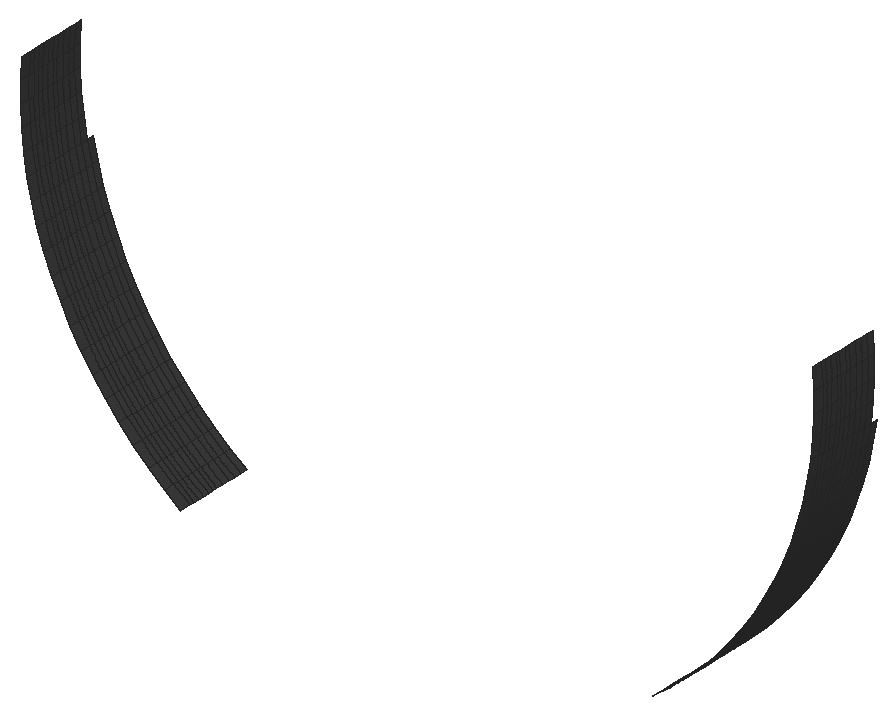
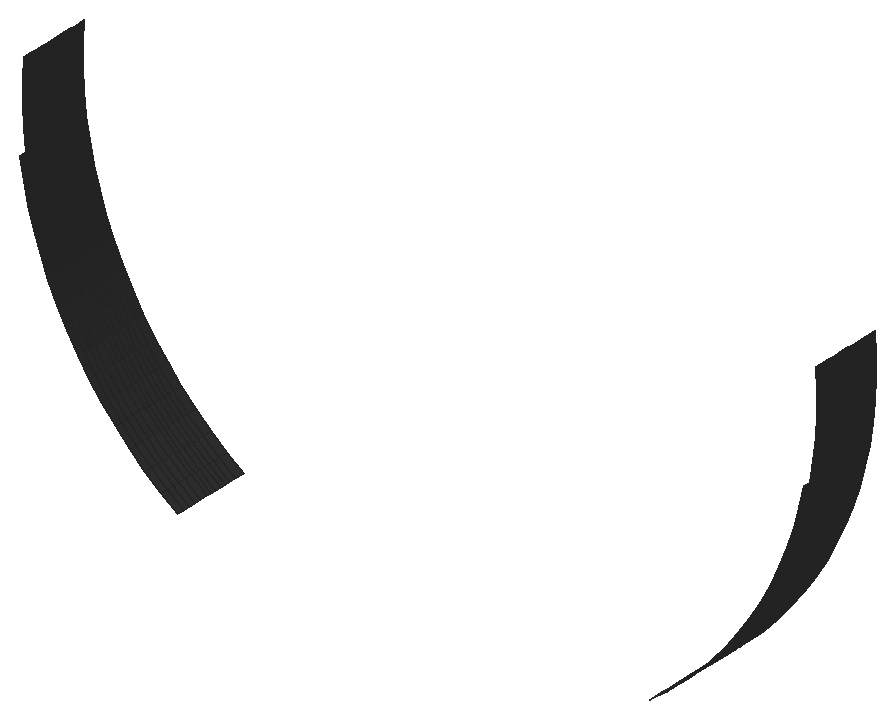
# SketchUp Ruby script. Lengths in inches.
U = 1.inch
M = Sketchup.active_model
def pt(a) = Geom::Point3d.new(a.map { |v| v * U })
def face(e, loops, mat)
  f = e.add_face(loops[0].map { |a| pt(a) })
  loops[1..].each { |l| e.add_face(l.map { |a| pt(a) }).erase! }
  f.material = f.back_material = mat if mat
  f
end
# faces: each face lists its corners as indices into pts; further lists are holes
def faces(e, pts, list, mat = nil) = list.each { |f| face(e, (f[0].is_a?(Array) ? f : [f]).map { |l| l.map { |i| pts[i] } }, mat) }
# xy, xz, yz: faces in a plane at the given z, y or x. An outline is a flat list of corners, or four numbers for a rectangle; further outlines are holes
def ring(l) = l.size == 4 ? [[l[0], l[1]], [l[2], l[1]], [l[2], l[3]], [l[0], l[3]]] : l.each_slice(2).to_a
def flat(e, list, mat, &to3) = list.each { |f| face(e, (f[0].is_a?(Array) ? f : [f]).map { |l| ring(l).map { |u, v| to3.(u, v) } }, mat) }
def xy(e, z, list, mat = nil) = flat(e, list, mat) { |x, y| [x, y, z] }
def xz(e, y, list, mat = nil) = flat(e, list, mat) { |x, z| [x, y, z] }
def yz(e, x, list, mat = nil) = flat(e, list, mat) { |y, z| [x, y, z] }
def lines(e, pts, list) = list.each { |a, b| e.add_line(pt(pts[a]), pt(pts[b])) }
# prism: a flat outline (further loops are holes) pulled along v
def prism(e, loops, v, mat = nil)
  f = face(e, loops, mat); d = Geom::Vector3d.new(v.map { |x| x * U })
  f.pushpull(f.normal.samedirection?(d) ? d.length : -d.length)
end
def box(e, o, s, mat = nil) = prism(e, [[o, [o[0] + s[0], o[1], o[2]], [o[0] + s[0], o[1] + s[1], o[2]], [o[0], o[1] + s[1], o[2]]]], [0, 0, s[2]], mat)
def at(x, y, z, deg = 0) = Geom::Transformation.translation(pt([x, y, z])) * Geom::Transformation.rotation(ORIGIN, Z_AXIS, deg.degrees)
def axes(o, x, y, z) = Geom::Transformation.new([*x, 0, *y, 0, *z, 0, *pt(o).to_a, 1])
def part(name) = M.definitions.add(name)
# library, detail: a bought-in or finely detailed component or shape, given as its bounding box
def library(name, o, s) = part(name).tap { |d| box(d.entities, o, s) }
def detail(e, o, s) = box(e.add_group.entities, o, s)
def put(e, d, t, mat = nil) = e.add_instance(d, t).tap { |i| i.material = mat if mat }
def group(e, t, mat = nil) = e.add_group.tap { |g| g.transformation = t; g.material = mat if mat }.entities
root = M.entities
M.materials.add("[Color M07]").color = [58, 58, 58]
yz(root,46.34,[[13.45,175.125,14.95,178.17],[14.95,175.125,15.8,178.17],[15.8,175.125,16.65,178.17],[16.65,175.125,17.5,178.17],[17.5,175.125,18.35,178.17],
  [18.35,175.125,19.21,178.17],[19.21,175.125,19.95,178.17],[19.95,175.125,21.02,178.17],[21.02,175.125,22.08,178.17],[22.08,175.125,23.14,178.17],
  [23.14,175.125,24.2,178.17]],"[Color M07]")
yz(root,160.49,[[13.45,175.125,14.95,178.17],[14.95,175.125,15.8,178.17],[15.8,175.125,16.65,178.17],[16.65,175.125,17.5,178.17],[17.5,175.125,18.35,178.17],
  [18.35,175.125,19.21,178.17],[19.21,175.125,19.95,178.17],[19.95,175.125,21.02,178.17],[21.02,175.125,22.08,178.17],[22.08,175.125,23.14,178.17],
  [23.14,175.125,24.2,178.17]],"[Color M07]")
p = [[69.46,13.45,130.82],[69.46,14.95,130.82],[67.06,14.95,132.69],[67.06,13.45,132.69],[139.77,13.45,132.69],[139.77,14.95,132.69],
  [137.375,14.95,130.82],[137.375,13.45,130.82],[69.46,15.8,130.82],[67.06,15.8,132.69],[139.77,15.8,132.69],[137.375,15.8,130.82],
  [69.46,16.65,130.82],[67.06,16.65,132.69],[139.77,16.65,132.69],[137.375,16.65,130.82],[69.46,17.5,130.82],[67.06,17.5,132.69],
  [139.77,17.5,132.69],[137.375,17.5,130.82],[69.46,18.35,130.82],[67.06,18.35,132.69],[139.77,18.35,132.69],[137.375,18.35,130.82],
  [69.46,19.21,130.82],[67.06,19.21,132.69],[139.77,19.21,132.69],[137.375,19.21,130.82],[69.46,19.95,130.82],[67.06,19.95,132.69],
  [139.77,19.95,132.69],[137.375,19.95,130.82],[69.46,21.02,130.82],[67.06,21.02,132.69],[139.77,21.02,132.69],[137.375,21.02,130.82],
  [69.46,22.08,130.82],[67.06,22.08,132.69],[139.77,22.08,132.69],[137.375,22.08,130.82],[69.46,23.14,130.82],[67.06,23.14,132.69],
  [139.77,23.14,132.69],[137.375,23.14,130.82],[69.46,24.2,130.82],[67.06,24.2,132.69],[139.77,24.2,132.69],[137.375,24.2,130.82],
  [69.46,25.27,130.82],[67.06,25.27,132.69],[139.77,25.27,132.69],[137.375,25.27,130.82],[64.77,14.95,134.69],[64.77,13.45,134.69],
  [142.0625,13.45,134.69],[142.0625,14.95,134.69],[64.77,15.8,134.69],[142.0625,15.8,134.69],[64.77,16.65,134.69],[142.0625,16.65,134.69],
  [64.77,17.5,134.69],[142.0625,17.5,134.69],[64.77,18.35,134.69],[142.0625,18.35,134.69],[64.77,19.21,134.69],[142.0625,19.21,134.69],
  [64.77,19.95,134.69],[142.0625,19.95,134.69],[64.77,21.02,134.69],[142.0625,21.02,134.69],[64.77,22.08,134.69],[142.0625,22.08,134.69],
  [64.77,23.14,134.69],[142.0625,23.14,134.69],[64.77,24.2,134.69],[142.0625,24.2,134.69],[64.77,25.27,134.69],[142.0625,25.27,134.69],
  [62.58,14.95,136.8125],[62.58,13.45,136.8125],[144.25,13.45,136.8125],[144.25,14.95,136.8125],[62.58,15.8,136.8125],[144.25,15.8,136.8125],
  [62.58,16.65,136.8125],[144.25,16.65,136.8125],[62.58,17.5,136.8125],[144.25,17.5,136.8125],[62.58,18.35,136.8125],[144.25,18.35,136.8125],
  [62.58,19.21,136.8125],[144.25,19.21,136.8125],[62.58,19.95,136.8125],[144.25,19.95,136.8125],[62.58,21.02,136.8125],[144.25,21.02,136.8125],
  [62.58,22.08,136.8125],[144.25,22.08,136.8125],[62.58,23.14,136.8125],[144.25,23.14,136.8125],[62.58,24.2,136.8125],[144.25,24.2,136.8125],
  [62.58,25.27,136.8125],[144.25,25.27,136.8125],[60.52,14.95,139.04],[60.52,13.45,139.04],[146.3125,13.45,139.04],[146.3125,14.95,139.04],
  [60.52,15.8,139.04],[146.3125,15.8,139.04],[60.52,16.65,139.04],[146.3125,16.65,139.04],[60.52,17.5,139.04],[146.3125,17.5,139.04],
  [60.52,18.35,139.04],[146.3125,18.35,139.04],[60.52,19.21,139.04],[146.3125,19.21,139.04],[60.52,19.95,139.04],[146.3125,19.95,139.04],
  [60.52,21.02,139.04],[146.3125,21.02,139.04],[60.52,22.08,139.04],[146.3125,22.08,139.04],[60.52,23.14,139.04],[146.3125,23.14,139.04],
  [60.52,24.2,139.04],[146.3125,24.2,139.04],[60.52,25.27,139.04],[146.3125,25.27,139.04],[58.57,14.95,141.38],[58.57,13.45,141.38],
  [148.26,13.45,141.38],[148.26,14.95,141.38],[58.57,15.8,141.38],[148.26,15.8,141.38],[58.57,16.65,141.38],[148.26,16.65,141.38],
  [58.57,17.5,141.38],[148.26,17.5,141.38],[58.57,18.35,141.38],[148.26,18.35,141.38],[58.57,19.21,141.38],[148.26,19.21,141.38],
  [58.57,19.95,141.38],[148.26,19.95,141.38],[58.57,21.02,141.38],[148.26,21.02,141.38],[58.57,22.08,141.38],[148.26,22.08,141.38],
  [58.57,23.14,141.38],[148.26,23.14,141.38],[58.57,24.2,141.38],[148.26,24.2,141.38],[58.57,25.27,141.38],[148.26,25.27,141.38],
  [56.75,14.95,143.82],[56.75,13.45,143.82],[150.08,13.45,143.82],[150.08,14.95,143.82],[56.75,15.8,143.82],[150.08,15.8,143.82],
  [56.75,16.65,143.82],[150.08,16.65,143.82],[56.75,17.5,143.82],[150.08,17.5,143.82],[56.75,18.35,143.82],[150.08,18.35,143.82],
  [56.75,19.21,143.82],[150.08,19.21,143.82],[56.75,19.95,143.82],[150.08,19.95,143.82],[56.75,21.02,143.82],[150.08,21.02,143.82],
  [56.75,22.08,143.82],[150.08,22.08,143.82],[56.75,23.14,143.82],[150.08,23.14,143.82],[56.75,24.2,143.82],[150.08,24.2,143.82],
  [56.75,25.27,143.82],[150.08,25.27,143.82],[55.07,14.95,146.35],[55.07,13.45,146.35],[151.76,13.45,146.35],[151.76,14.95,146.35],
  [55.07,15.8,146.35],[151.76,15.8,146.35],[55.07,16.65,146.35],[151.76,16.65,146.35],[55.07,17.5,146.35],[151.76,17.5,146.35],
  [55.07,18.35,146.35],[151.76,18.35,146.35],[55.07,19.21,146.35],[151.76,19.21,146.35],[55.07,19.95,146.35],[151.76,19.95,146.35],
  [55.07,21.02,146.35],[151.76,21.02,146.35],[55.07,22.08,146.35],[151.76,22.08,146.35],[55.07,23.14,146.35],[151.76,23.14,146.35],
  [55.07,24.2,146.35],[151.76,24.2,146.35],[55.07,25.27,146.35],[151.76,25.27,146.35],[53.52,14.95,148.97],[53.52,13.45,148.97],
  [153.3125,13.45,148.97],[153.3125,14.95,148.97],[53.52,15.8,148.97],[153.3125,15.8,148.97],[53.52,16.65,148.97],[153.3125,16.65,148.97],
  [53.52,17.5,148.97],[153.3125,17.5,148.97],[53.52,18.35,148.97],[153.3125,18.35,148.97],[53.52,19.21,148.97],[153.3125,19.21,148.97],
  [53.52,19.95,148.97],[153.3125,19.95,148.97],[53.52,21.02,148.97],[153.3125,21.02,148.97],[53.52,22.08,148.97],[153.3125,22.08,148.97],
  [53.52,23.14,148.97],[153.3125,23.14,148.97],[53.52,24.2,148.97],[153.3125,24.2,148.97],[53.52,25.27,148.97],[153.3125,25.27,148.97],
  [52.11,14.95,151.67],[52.11,13.45,151.67],[154.72,13.45,151.67],[154.72,14.95,151.67],[52.11,15.8,151.67],[154.72,15.8,151.67],
  [52.11,16.65,151.67],[154.72,16.65,151.67],[52.11,17.5,151.67],[154.72,17.5,151.67],[52.11,18.35,151.67],[154.72,18.35,151.67],
  [52.11,19.21,151.67],[154.72,19.21,151.67],[52.11,19.95,151.67],[154.72,19.95,151.67],[52.11,21.02,151.67],[154.72,21.02,151.67],
  [52.11,22.08,151.67],[154.72,22.08,151.67],[52.11,23.14,151.67],[154.72,23.14,151.67],[52.11,24.2,151.67],[154.72,24.2,151.67],
  [52.11,25.27,151.67],[154.72,25.27,151.67],[50.85,14.95,154.4375],[50.85,13.45,154.4375],[155.98,13.45,154.4375],[155.98,14.95,154.4375],
  [50.85,15.8,154.4375],[155.98,15.8,154.4375],[50.85,16.65,154.4375],[155.98,16.65,154.4375],[50.85,17.5,154.4375],[155.98,17.5,154.4375],
  [50.85,18.35,154.4375],[155.98,18.35,154.4375],[50.85,19.21,154.4375],[155.98,19.21,154.4375],[50.85,19.95,154.4375],[155.98,19.95,154.4375],
  [50.85,21.02,154.4375],[155.98,21.02,154.4375],[50.85,22.08,154.4375],[155.98,22.08,154.4375],[50.85,23.14,154.4375],[155.98,23.14,154.4375],
  [50.85,24.2,154.4375],[155.98,24.2,154.4375],[50.85,25.27,154.4375],[155.98,25.27,154.4375],[49.74,14.95,157.27],[49.74,13.45,157.27],
  [157.09,13.45,157.27],[157.09,14.95,157.27],[49.74,15.8,157.27],[157.09,15.8,157.27],[49.74,16.65,157.27],[157.09,16.65,157.27],
  [49.74,17.5,157.27],[157.09,17.5,157.27],[49.74,18.35,157.27],[157.09,18.35,157.27],[49.74,19.21,157.27],[157.09,19.21,157.27],
  [49.74,19.95,157.27],[157.09,19.95,157.27],[49.74,21.02,157.27],[157.09,21.02,157.27],[49.74,22.08,157.27],[157.09,22.08,157.27],
  [49.74,23.14,157.27],[157.09,23.14,157.27],[49.74,24.2,157.27],[157.09,24.2,157.27],[49.74,25.27,157.27],[157.09,25.27,157.27],
  [48.78,14.95,160.15],[48.78,13.45,160.15],[158.05,13.45,160.15],[158.05,14.95,160.15],[48.78,15.8,160.15],[158.05,15.8,160.15],
  [48.78,16.65,160.15],[158.05,16.65,160.15],[48.78,17.5,160.15],[158.05,17.5,160.15],[48.78,18.35,160.15],[158.05,18.35,160.15],
  [48.78,19.21,160.15],[158.05,19.21,160.15],[48.78,19.95,160.15],[158.05,19.95,160.15],[48.78,21.02,160.15],[158.05,21.02,160.15],
  [48.78,22.08,160.15],[158.05,22.08,160.15],[48.78,23.14,160.15],[158.05,23.14,160.15],[48.78,24.2,160.15],[158.05,24.2,160.15],
  [48.78,25.27,160.15],[158.05,25.27,160.15],[47.97,14.95,163.09],[47.97,13.45,163.09],[158.86,13.45,163.09],[158.86,14.95,163.09],
  [47.97,15.8,163.09],[158.86,15.8,163.09],[47.97,16.65,163.09],[158.86,16.65,163.09],[47.97,17.5,163.09],[158.86,17.5,163.09],
  [47.97,18.35,163.09],[158.86,18.35,163.09],[47.97,19.21,163.09],[158.86,19.21,163.09],[47.97,19.95,163.09],[158.86,19.95,163.09],
  [47.97,21.02,163.09],[158.86,21.02,163.09],[47.97,22.08,163.09],[158.86,22.08,163.09],[47.97,23.14,163.09],[158.86,23.14,163.09],
  [47.97,24.2,163.09],[158.86,24.2,163.09],[47.97,25.27,163.09],[158.86,25.27,163.09],[47.32,14.95,166.0625],[47.32,13.45,166.0625],
  [159.51,13.45,166.0625],[159.51,14.95,166.0625],[47.32,15.8,166.0625],[159.51,15.8,166.0625],[47.32,16.65,166.0625],[159.51,16.65,166.0625],
  [47.32,17.5,166.0625],[159.51,17.5,166.0625],[47.32,18.35,166.0625],[159.51,18.35,166.0625],[47.32,19.21,166.0625],[159.51,19.21,166.0625],
  [47.32,19.95,166.0625],[159.51,19.95,166.0625],[47.32,21.02,166.0625],[159.51,21.02,166.0625],[47.32,22.08,166.0625],[159.51,22.08,166.0625],
  [47.32,23.14,166.0625],[159.51,23.14,166.0625],[47.32,24.2,166.0625],[159.51,24.2,166.0625],[47.32,25.27,166.0625],[159.51,25.27,166.0625],
  [46.84,14.95,169.0625],[46.84,13.45,169.0625],[159.99,13.45,169.0625],[159.99,14.95,169.0625],[46.84,15.8,169.0625],[159.99,15.8,169.0625],
  [46.84,16.65,169.0625],[159.99,16.65,169.0625],[46.84,17.5,169.0625],[159.99,17.5,169.0625],[46.84,18.35,169.0625],[159.99,18.35,169.0625],
  [46.84,19.21,169.0625],[159.99,19.21,169.0625],[46.84,19.95,169.0625],[159.99,19.95,169.0625],[46.84,21.02,169.0625],[159.99,21.02,169.0625],
  [46.84,22.08,169.0625],[159.99,22.08,169.0625],[46.84,23.14,169.0625],[159.99,23.14,169.0625],[46.84,24.2,169.0625],[159.99,24.2,169.0625],
  [159.99,25.27,169.0625],[46.51,14.95,172.09],[46.51,13.45,172.09],[160.32,13.45,172.09],[160.32,14.95,172.09],[46.51,15.8,172.09],
  [160.32,15.8,172.09],[46.51,16.65,172.09],[160.32,16.65,172.09],[46.51,17.5,172.09],[160.32,17.5,172.09],[46.51,18.35,172.09],
  [160.32,18.35,172.09],[46.51,19.21,172.09],[160.32,19.21,172.09],[46.51,19.95,172.09],[160.32,19.95,172.09],[46.51,21.02,172.09],
  [160.32,21.02,172.09],[46.51,22.08,172.09],[160.32,22.08,172.09],[46.51,23.14,172.09],[160.32,23.14,172.09],[46.51,24.2,172.09],
  [160.32,24.2,172.09],[46.34,14.95,175.125],[46.34,13.45,175.125],[160.49,13.45,175.125],[160.49,14.95,175.125],[46.34,15.8,175.125],
  [160.49,15.8,175.125],[46.34,16.65,175.125],[160.49,16.65,175.125],[46.34,17.5,175.125],[160.49,17.5,175.125],[46.34,18.35,175.125],
  [160.49,18.35,175.125],[46.34,19.21,175.125],[160.49,19.21,175.125],[46.34,19.95,175.125],[160.49,19.95,175.125],[46.34,21.02,175.125],
  [160.49,21.02,175.125],[46.34,22.08,175.125],[160.49,22.08,175.125],[46.34,23.14,175.125],[160.49,23.14,175.125],[46.34,24.2,175.125],
  [160.49,24.2,175.125],[46.34,13.45,178.17],[46.34,14.95,178.17],[46.5,14.95,181.21],[46.5,13.45,181.21],[160.33,13.45,181.21],
  [160.33,14.95,181.21],[160.49,14.95,178.17],[160.49,13.45,178.17],[46.34,15.8,178.17],[46.5,15.8,181.21],[160.33,15.8,181.21],
  [160.49,15.8,178.17],[46.34,16.65,178.17],[46.5,16.65,181.21],[160.33,16.65,181.21],[160.49,16.65,178.17],[46.34,17.5,178.17],
  [46.5,17.5,181.21],[160.33,17.5,181.21],[160.49,17.5,178.17],[46.34,18.35,178.17],[46.5,18.35,181.21],[160.33,18.35,181.21],
  [160.49,18.35,178.17],[46.34,19.21,178.17],[46.5,19.21,181.21],[160.33,19.21,181.21],[160.49,19.21,178.17],[46.34,19.95,178.17],
  [46.5,19.95,181.21],[160.33,19.95,181.21],[160.49,19.95,178.17],[46.34,21.02,178.17],[46.5,21.02,181.21],[160.33,21.02,181.21],
  [160.49,21.02,178.17],[46.34,22.08,178.17],[46.5,22.08,181.21],[160.33,22.08,181.21],[160.49,22.08,178.17],[46.34,23.14,178.17],
  [46.5,23.14,181.21],[160.33,23.14,181.21],[160.49,23.14,178.17],[46.34,24.2,178.17],[46.5,24.2,181.21],[160.33,24.2,181.21],
  [160.49,24.2,178.17]]
faces(root,p,[[0,1,2,3],[4,5,6,7],[1,8,9,2],[5,10,11,6],[8,12,13,9],[10,14,15,11],[12,16,17,13],[14,18,19,15],
  [16,20,21,17],[18,22,23,19],[20,24,25,21],[22,26,27,23],[24,28,29,25],[26,30,31,27],[28,32,33,29],[30,34,35,31],
  [32,36,37,33],[34,38,39,35],[36,40,41,37],[38,42,43,39],[40,44,45,41],[42,46,47,43],[44,48,49,45],[46,50,51,47],
  [3,2,52,53],[54,55,5,4],[2,9,56,52],[55,57,10,5],[9,13,58,56],[57,59,14,10],[13,17,60,58],[59,61,18,14],
  [17,21,62,60],[61,63,22,18],[21,25,64,62],[63,65,26,22],[25,29,66,64],[65,67,30,26],[29,33,68,66],[67,69,34,30],
  [33,37,70,68],[69,71,38,34],[37,41,72,70],[71,73,42,38],[41,45,74,72],[73,75,46,42],[45,49,76,74],[75,77,50,46],
  [53,52,78,79],[80,81,55,54],[52,56,82,78],[81,83,57,55],[56,58,84,82],[83,85,59,57],[58,60,86,84],[85,87,61,59],
  [60,62,88,86],[87,89,63,61],[62,64,90,88],[89,91,65,63],[64,66,92,90],[91,93,67,65],[66,68,94,92],[93,95,69,67],
  [68,70,96,94],[95,97,71,69],[70,72,98,96],[97,99,73,71],[72,74,100,98],[99,101,75,73],[74,76,102,100],[101,103,77,75],
  [79,78,104,105],[106,107,81,80],[78,82,108,104],[107,109,83,81],[82,84,110,108],[109,111,85,83],[84,86,112,110],[111,113,87,85],
  [86,88,114,112],[113,115,89,87],[88,90,116,114],[115,117,91,89],[90,92,118,116],[117,119,93,91],[92,94,120,118],[119,121,95,93],
  [94,96,122,120],[121,123,97,95],[96,98,124,122],[123,125,99,97],[98,100,126,124],[125,127,101,99],[100,102,128,126],[127,129,103,101],
  [105,104,130,131],[132,133,107,106],[104,108,134,130],[133,135,109,107],[108,110,136,134],[135,137,111,109],[110,112,138,136],[137,139,113,111],
  [112,114,140,138],[139,141,115,113],[114,116,142,140],[141,143,117,115],[116,118,144,142],[143,145,119,117],[118,120,146,144],[145,147,121,119],
  [120,122,148,146],[147,149,123,121],[122,124,150,148],[149,151,125,123],[124,126,152,150],[151,153,127,125],[126,128,154,152],[153,155,129,127],
  [131,130,156,157],[158,159,133,132],[130,134,160,156],[159,161,135,133],[134,136,162,160],[161,163,137,135],[136,138,164,162],[163,165,139,137],
  [138,140,166,164],[165,167,141,139],[140,142,168,166],[167,169,143,141],[142,144,170,168],[169,171,145,143],[144,146,172,170],[171,173,147,145],
  [146,148,174,172],[173,175,149,147],[148,150,176,174],[175,177,151,149],[150,152,178,176],[177,179,153,151],[152,154,180,178],[179,181,155,153],
  [157,156,182,183],[184,185,159,158],[156,160,186,182],[185,187,161,159],[160,162,188,186],[187,189,163,161],[162,164,190,188],[189,191,165,163],
  [164,166,192,190],[191,193,167,165],[166,168,194,192],[193,195,169,167],[168,170,196,194],[195,197,171,169],[170,172,198,196],[197,199,173,171],
  [172,174,200,198],[199,201,175,173],[174,176,202,200],[201,203,177,175],[176,178,204,202],[203,205,179,177],[178,180,206,204],[205,207,181,179],
  [183,182,208,209],[210,211,185,184],[182,186,212,208],[211,213,187,185],[186,188,214,212],[213,215,189,187],[188,190,216,214],[215,217,191,189],
  [190,192,218,216],[217,219,193,191],[192,194,220,218],[219,221,195,193],[194,196,222,220],[221,223,197,195],[196,198,224,222],[223,225,199,197],
  [198,200,226,224],[225,227,201,199],[200,202,228,226],[227,229,203,201],[202,204,230,228],[229,231,205,203],[204,206,232,230],[231,233,207,205],
  [209,208,234,235],[236,237,211,210],[208,212,238,234],[237,239,213,211],[212,214,240,238],[239,241,215,213],[214,216,242,240],[241,243,217,215],
  [216,218,244,242],[243,245,219,217],[218,220,246,244],[245,247,221,219],[220,222,248,246],[247,249,223,221],[222,224,250,248],[249,251,225,223],
  [224,226,252,250],[251,253,227,225],[226,228,254,252],[253,255,229,227],[228,230,256,254],[255,257,231,229],[230,232,258,256],[257,259,233,231],
  [235,234,260,261],[262,263,237,236],[234,238,264,260],[263,265,239,237],[238,240,266,264],[265,267,241,239],[240,242,268,266],[267,269,243,241],
  [242,244,270,268],[269,271,245,243],[244,246,272,270],[271,273,247,245],[246,248,274,272],[273,275,249,247],[248,250,276,274],[275,277,251,249],
  [250,252,278,276],[277,279,253,251],[252,254,280,278],[279,281,255,253],[254,256,282,280],[281,283,257,255],[256,258,284,282],[283,285,259,257],
  [261,260,286,287],[288,289,263,262],[260,264,290,286],[289,291,265,263],[264,266,292,290],[291,293,267,265],[266,268,294,292],[293,295,269,267],
  [268,270,296,294],[295,297,271,269],[270,272,298,296],[297,299,273,271],[272,274,300,298],[299,301,275,273],[274,276,302,300],[301,303,277,275],
  [276,278,304,302],[303,305,279,277],[278,280,306,304],[305,307,281,279],[280,282,308,306],[307,309,283,281],[282,284,310,308],[309,311,285,283],
  [287,286,312,313],[314,315,289,288],[286,290,316,312],[315,317,291,289],[290,292,318,316],[317,319,293,291],[292,294,320,318],[319,321,295,293],
  [294,296,322,320],[321,323,297,295],[296,298,324,322],[323,325,299,297],[298,300,326,324],[325,327,301,299],[300,302,328,326],[327,329,303,301],
  [302,304,330,328],[329,331,305,303],[304,306,332,330],[331,333,307,305],[306,308,334,332],[333,335,309,307],[308,310,336,334],[335,337,311,309],
  [313,312,338,339],[340,341,315,314],[312,316,342,338],[341,343,317,315],[316,318,344,342],[343,345,319,317],[318,320,346,344],[345,347,321,319],
  [320,322,348,346],[347,349,323,321],[322,324,350,348],[349,351,325,323],[324,326,352,350],[351,353,327,325],[326,328,354,352],[353,355,329,327],
  [328,330,356,354],[355,357,331,329],[330,332,358,356],[357,359,333,331],[332,334,360,358],[359,361,335,333],[334,336,362,360],[361,363,337,335],
  [339,338,364,365],[366,367,341,340],[338,342,368,364],[367,369,343,341],[342,344,370,368],[369,371,345,343],[344,346,372,370],[371,373,347,345],
  [346,348,374,372],[373,375,349,347],[348,350,376,374],[375,377,351,349],[350,352,378,376],[377,379,353,351],[352,354,380,378],[379,381,355,353],
  [354,356,382,380],[381,383,357,355],[356,358,384,382],[383,385,359,357],[358,360,386,384],[385,387,361,359],[360,362,388,386],[387,389,363,361],
  [365,364,390,391],[392,393,367,366],[364,368,394,390],[393,395,369,367],[368,370,396,394],[395,397,371,369],[370,372,398,396],[397,399,373,371],
  [372,374,400,398],[399,401,375,373],[374,376,402,400],[401,403,377,375],[376,378,404,402],[403,405,379,377],[378,380,406,404],[405,407,381,379],
  [380,382,408,406],[407,409,383,381],[382,384,410,408],[409,411,385,383],[384,386,412,410],[411,413,387,385],[413,414,389,387],[391,390,415,416],
  [417,418,393,392],[390,394,419,415],[418,420,395,393],[394,396,421,419],[420,422,397,395],[396,398,423,421],[422,424,399,397],[398,400,425,423],
  [424,426,401,399],[400,402,427,425],[426,428,403,401],[402,404,429,427],[428,430,405,403],[404,406,431,429],[430,432,407,405],[406,408,433,431],
  [432,434,409,407],[408,410,435,433],[434,436,411,409],[410,412,437,435],[436,438,413,411],[416,415,439,440],[441,442,418,417],[415,419,443,439],
  [442,444,420,418],[419,421,445,443],[444,446,422,420],[421,423,447,445],[446,448,424,422],[423,425,449,447],[448,450,426,424],[425,427,451,449],
  [450,452,428,426],[427,429,453,451],[452,454,430,428],[429,431,455,453],[454,456,432,430],[431,433,457,455],[456,458,434,432],[433,435,459,457],
  [458,460,436,434],[435,437,461,459],[460,462,438,436],[463,464,465,466],[467,468,469,470],[464,471,472,465],[468,473,474,469],[471,475,476,472],
  [473,477,478,474],[475,479,480,476],[477,481,482,478],[479,483,484,480],[481,485,486,482],[483,487,488,484],[485,489,490,486],[487,491,492,488],
  [489,493,494,490],[491,495,496,492],[493,497,498,494],[495,499,500,496],[497,501,502,498],[499,503,504,500],[501,505,506,502],[503,507,508,504],
  [505,509,510,506]],"[Color M07]")
